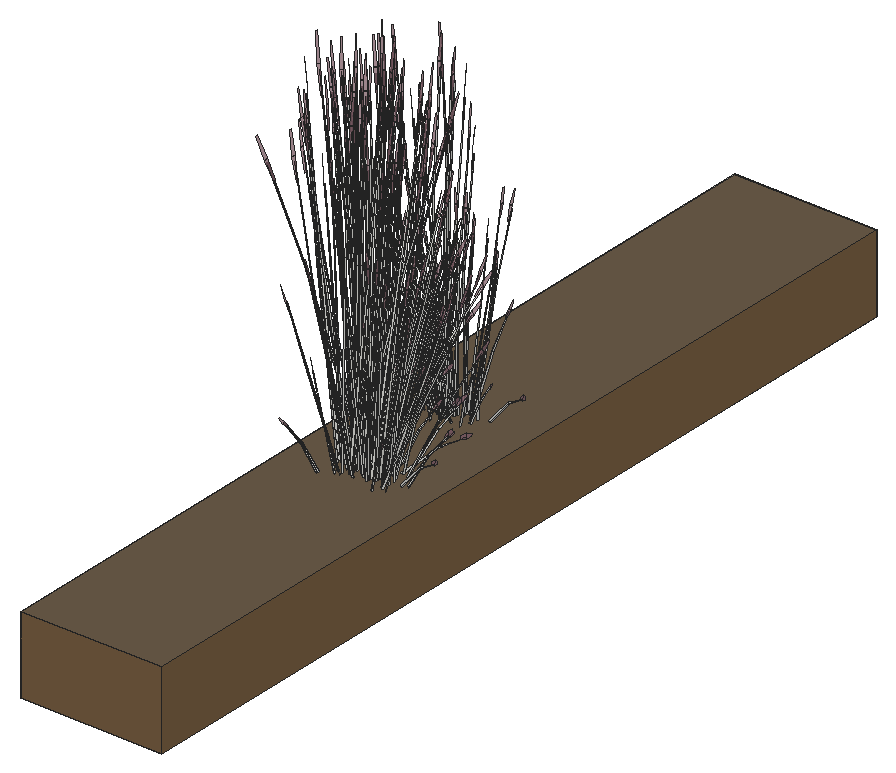
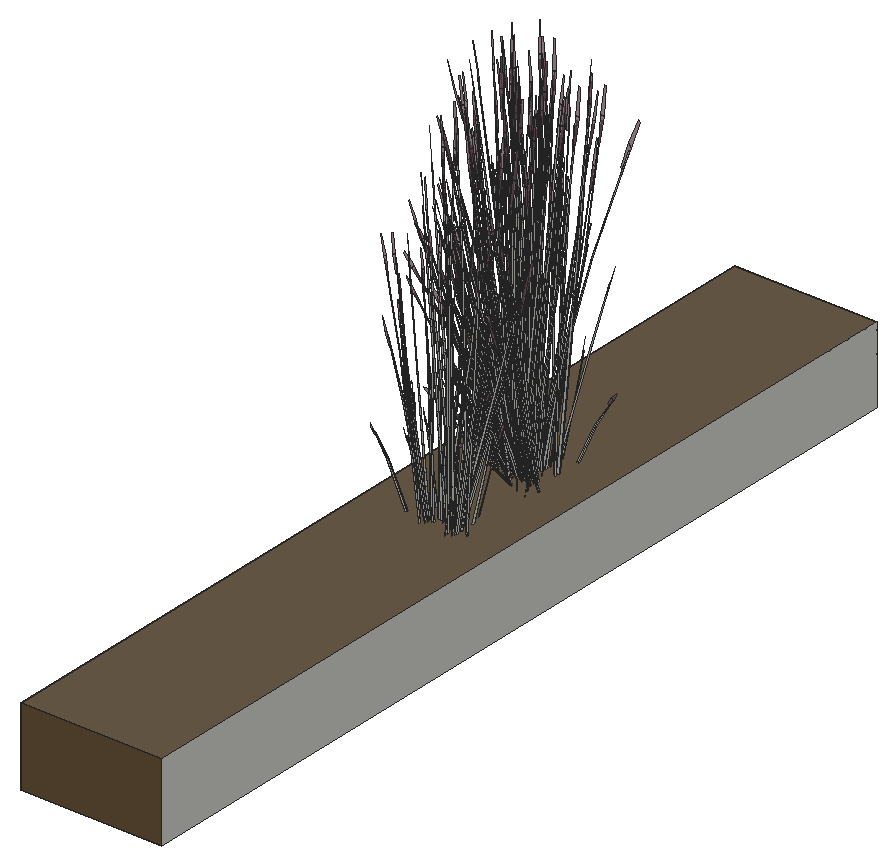
# SketchUp Ruby script. Lengths in inches.
U = 1.inch
M = Sketchup.active_model
def pt(a) = Geom::Point3d.new(a.map { |v| v * U })
def face(e, loops, mat)
  f = e.add_face(loops[0].map { |a| pt(a) })
  loops[1..].each { |l| e.add_face(l.map { |a| pt(a) }).erase! }
  f.material = f.back_material = mat if mat
  f
end
# faces: each face lists its corners as indices into pts; further lists are holes
def faces(e, pts, list, mat = nil) = list.each { |f| face(e, (f[0].is_a?(Array) ? f : [f]).map { |l| l.map { |i| pts[i] } }, mat) }
# xy, xz, yz: faces in a plane at the given z, y or x. An outline is a flat list of corners, or four numbers for a rectangle; further outlines are holes
def ring(l) = l.size == 4 ? [[l[0], l[1]], [l[2], l[1]], [l[2], l[3]], [l[0], l[3]]] : l.each_slice(2).to_a
def flat(e, list, mat, &to3) = list.each { |f| face(e, (f[0].is_a?(Array) ? f : [f]).map { |l| ring(l).map { |u, v| to3.(u, v) } }, mat) }
def xy(e, z, list, mat = nil) = flat(e, list, mat) { |x, y| [x, y, z] }
def xz(e, y, list, mat = nil) = flat(e, list, mat) { |x, z| [x, y, z] }
def yz(e, x, list, mat = nil) = flat(e, list, mat) { |y, z| [x, y, z] }
def lines(e, pts, list) = list.each { |a, b| e.add_line(pt(pts[a]), pt(pts[b])) }
# prism: a flat outline (further loops are holes) pulled along v
def prism(e, loops, v, mat = nil)
  f = face(e, loops, mat); d = Geom::Vector3d.new(v.map { |x| x * U })
  f.pushpull(f.normal.samedirection?(d) ? d.length : -d.length)
end
def box(e, o, s, mat = nil) = prism(e, [[o, [o[0] + s[0], o[1], o[2]], [o[0] + s[0], o[1] + s[1], o[2]], [o[0], o[1] + s[1], o[2]]]], [0, 0, s[2]], mat)
def at(x, y, z, deg = 0) = Geom::Transformation.translation(pt([x, y, z])) * Geom::Transformation.rotation(ORIGIN, Z_AXIS, deg.degrees)
def axes(o, x, y, z) = Geom::Transformation.new([*x, 0, *y, 0, *z, 0, *pt(o).to_a, 1])
def part(name) = M.definitions.add(name)
# library, detail: a bought-in or finely detailed component or shape, given as its bounding box
def library(name, o, s) = part(name).tap { |d| box(d.entities, o, s) }
def detail(e, o, s) = box(e.add_group.entities, o, s)
def put(e, d, t, mat = nil) = e.add_instance(d, t).tap { |i| i.material = mat if mat }
def group(e, t, mat = nil) = e.add_group.tap { |g| g.transformation = t; g.material = mat if mat }.entities
root = M.entities
M.materials.add("Forest_Floor_01_1K").color = [106, 91, 72]
M.materials.add("LightPink_Translucent").color = [144, 107, 117]
M.materials["LightPink_Translucent"].alpha = 0.75
M.materials.add("Soil_03_1K").color = [122, 96, 67]
c1 = part("blade")
p = [[2.15,0.21,22],[0,0.17,0],[0.09,0.45,0],[2.18,0.31,22],[2.29,0.31,22],[0.38,0.45,0],
  [2.48,0.24,33],[2.49,0.24,33],[2.48,0.22,33]]
faces(c1.entities,p,[[0,1,2,3],[4,5,2,3],[6,3,4,7],[8,0,3,6]])
c2 = part("seeds")
p = [[0.3,-0.1,1.38],[-0.01,-0.03,1.59],[-0.01,-0.03,0.03],[0.14,-0.07,-0.07],[0.29,-0.03,3],[0.15,0.01,3.11]]
faces(c2.entities,p,[[0,1,2,3],[1,0,4,5]],"LightPink_Translucent")
c3 = part("blade with seeds")
put(c3.entities,c1,at(0,0,0))
put(c3.entities,c2,axes([2.4,0.25,30.99],[1.5799,-0.05474,1.17369],[-0.12525,1.92788,0.29478],[-0.07173,-0.02425,1.56792]))
xy(root,-6,[[498.15,426.77,519.85,563.22]])
xy(root,5.86,[[498.15,426.77,519.85,563.22]],"Forest_Floor_01_1K")
xz(root,426.77,[[498.15,-6,519.85,5.86]],"Soil_03_1K")
xz(root,563.22,[[498.15,-6,519.85,5.86]],"Soil_03_1K")
yz(root,498.15,[[426.77,-6,563.22,5.86]])
yz(root,519.85,[[426.77,-6,563.22,5.86]],"Soil_03_1K")
put(root,c3,axes([510.03,477.89,3.72],[0.5141,-0.32171,-0.35414],[0.48666,0.36734,0.4572],[0.07405,-0.18664,0.87481]))
put(root,c3,axes([505.58,476.76,1.96],[0.39634,0.21267,1.1486],[-0.57721,0.12784,0.84392],[-0.1235,-0.16344,0.25299]))
put(root,c3,axes([508.52,477.39,3.92],[0.55987,-0.20767,0.0643],[0.27403,0.37869,0.50621],[-0.05407,-0.16693,0.77189]))
put(root,c3,axes([506.61,477.45,3.92],[0.34533,-0.38816,0.0643],[0.49176,0.22599,0.50621],[-0.15898,-0.12445,0.77189]))
put(root,c3,axes([506.5,479.61,1.29],[-0.31203,-0.62659,-0.69835],[0.89884,-0.22566,-0.18329],[-0.03449,-0.21218,1.54149]))
put(root,c3,axes([510.67,477.7,0.6875],[-0.11372,-0.04814,1.76342],[-0.29211,-0.53779,-0.26939],[0.19706,-0.14594,0.30037]))
put(root,c3,axes([508.32,477.82,4.24],[-0.22906,0.4699,0.35414],[-0.66828,-0.13705,-0.4572],[-0.06128,-0.18919,0.87481]))
put(root,c3,axes([510.03,478.02,3.93],[0.54105,0.41691,0.48003],[-0.57458,0.35956,0.3958],[0.0998,-0.1956,0.9933]))
put(root,c3,axes([510.22,478.06,3.92],[0.62439,0.02847,0.0643],[-0.01712,0.42991,0.50621],[0.06534,-0.16468,0.77189]))
put(root,c3,axes([509.76,478.35,4.24],[-0.5141,0.32171,0.35414],[-0.48666,-0.36734,-0.4572],[0.07405,-0.18664,0.87481]))
put(root,c3,axes([510.67,479.22,4.17],[0.39688,-0.48213,-0.71045],[0.69548,0.34264,0.08574],[0.23697,-0.17468,1.00501]))
put(root,c3,axes([506.375,477.8125,1.57],[-0.47504,-0.61229,0],[0.79476,-0.34146,-0.51607],[0.18101,-0.07777,1.63711]))
put(root,c3,axes([510.65,478.99,3.875],[-0.19519,-0.55794,-0.51099],[0.73919,-0.0976,-0.3958],[0.21183,-0.14986,0.97773]))
put(root,c3,axes([507.42,477.07,1.32],[-0.52505,0.35054,-0.03893],[-0.48109,-0.38392,-0.17649],[-0.03387,-0.10878,0.58215]))
put(root,c3,axes([510.99,479.39,4.23],[-0.70283,-0.33692,-0.1216],[0.40491,-0.48793,-0.67495],[0.19857,-0.16961,1.02557]))
put(root,c3,axes([508.09,481.23,2.52],[0.65659,0.2464,1.51261],[-0.64324,0.53082,0.59816],[-0.28812,-0.31461,1.26806]))
put(root,c3,axes([504.66,479.53,1.21],[0,-0.61104,-0.49651],[0.85008,0,0],[0,-0.13917,1.57504]))
put(root,c3,axes([507.02,477.72,1.21],[0.7111,-0.30552,-0.49651],[0.42504,0.54784,0],[0.16196,-0.06958,1.57504]))
put(root,c3,axes([511.24,478.77,1.78],[-0.27143,-0.0181,1.43002],[-0.27808,-0.48551,-0.30754],[0.33346,-0.13735,0.61141]))
put(root,c3,axes([512.72,479.24,3.9],[-0.09924,-0.00464,1.77383],[-0.4121,-0.49725,-0.16761],[0.1655,-0.1635,0.31391]))
put(root,c3,axes([507.86,478.97,1.25],[0.51177,-0.45928,-0.62353],[0.63575,0.41646,-0.16365],[0.20507,-0.11457,1.37633]))
put(root,c3,axes([511.55,477.88,1.96],[-0.25308,0.31105,1.1486],[-0.21753,-0.4179,0.84392],[0.20902,-0.10472,0.25299]))
put(root,c3,axes([511.19,479.05,3.72],[0.66138,-0.08733,-0.35414],[0.17464,0.49921,0.4572],[0.18953,-0.13408,0.87481]))
put(root,c3,axes([506.97,479.78,1.4],[0.36864,-0.55059,-0.44739],[0.76598,0.26498,0.21531],[0,-0.12692,1.43643]))
put(root,c3,axes([507.31,479.5,1.86],[-0.08854,-0.69723,-0.29095],[0.92215,-0.04216,-0.50002],[0.16238,-0.09287,1.59708]))
put(root,c3,axes([505.02,479.54,1.22],[0.53038,-0.38124,-0.30978],[0.53038,0.38124,0.30978],[0,-0.1228,1.38974]))
put(root,c3,axes([510.65,479.34,4.24],[-0.66138,0.08733,0.35414],[-0.17464,-0.49921,-0.4572],[0.18953,-0.13408,0.87481]))
put(root,c3,axes([506.88,480.23,1.86],[-0.85568,-0.29155,-0.29095],[0.41201,-0.61537,-0.50002],[-0.02689,-0.15109,1.59708]))
put(root,c3,axes([507.1875,477.96,1.22],[0.70886,0.15119,-0.30978],[-0.17848,0.53243,0.30978],[0.1429,-0.0614,1.38974]))
put(root,c3,axes([511.25,479.27,3.92],[0.52161,0.25698,0.0643],[-0.30368,0.36595,0.50621],[0.16723,-0.11831,0.77189]))
put(root,c3,axes([511.11,479.16,3.93],[0.18844,0.56237,0.48003],[-0.73919,0.0976,0.3958],[0.21785,-0.13226,0.9933]))
put(root,c3,axes([513.1,479.84,3.91],[0.10543,-0.09307,1.74944],[-0.13495,-0.57092,-0.27667],[0.26455,-0.10825,0.14031]))
put(root,c3,axes([505.18,479.81,1.52],[-0.70674,0.51372,0.30756],[-0.70717,-0.50832,-0.36492],[-0.02468,-0.14589,1.64885]))
put(root,c3,axes([507.43,480.05,1.625],[0.8561,0.29616,0.24065],[-0.41201,0.61537,0.50002],[0,-0.14185,1.60543]))
put(root,c3,axes([507.1,480.88,1.63],[0.20138,-0.72405,-0.23429],[0.95485,0.12621,0.51271],[-0.16685,-0.09999,1.5644]))
put(root,c3,axes([507.15,479.64,1.91],[-0.82508,0.03772,0.44739],[-0.07462,-0.62614,-0.21531],[0.14771,-0.06346,1.43643]))
put(root,c3,axes([505.02,480.09,1.67],[0,0.61104,0.49651],[-0.85008,0,0],[0,-0.13917,1.57504]))
put(root,c3,axes([511.02,480.71,4.23],[-0.38229,-0.5533,-0.1216],[0.6785,-0.2719,-0.67495],[0.28593,-0.073,1.02557]))
put(root,c3,axes([510.99,480.23,3.875],[0.20584,-0.55581,-0.51099],[0.70573,0.19051,-0.3958],[0.28414,-0.05097,0.97773]))
put(root,c3,axes([509.875,477.97,1.57],[0.47504,-0.61229,0],[0.79476,0.34146,-0.51607],[0.18101,0.07777,1.63711]))
put(root,c3,axes([507.03,480.59,1.4],[-0.45644,-0.51287,-0.44739],[0.69137,-0.36116,0.21531],[-0.14771,-0.06346,1.43643]))
put(root,c3,axes([507.125,479.86,1.55],[0.33034,0.68327,0.45755],[-0.94388,0.2376,0.17955],[0.01154,-0.12555,1.58856]))
put(root,c3,axes([511.74,480.39,1.17],[-0.48937,0.07333,1.41583],[-0.07789,-0.58369,0.08104],[0.34275,-0.08835,0.80566]))
put(root,c3,axes([512.63,479.87,1.45],[-0.47106,-0.39072,-0.06488],[0.51591,-0.35801,-0.29416],[0.14618,-0.02521,0.97024]))
put(root,c3,axes([506.96,480.4,1.91],[-0.36864,0.55059,0.44739],[-0.76598,-0.26498,-0.21531],[0,-0.12692,1.43643]))
put(root,c3,axes([508.3125,479.92,1.4],[0,-0.70701,0],[0.95008,0,0],[0,0,1.79456]))
put(root,c3,axes([509.46,478.29,1.67],[-0.7111,-0.30552,0.49651],[0.42504,-0.54784,0],[0.16196,0.06958,1.57504]))
put(root,c3,axes([510.85,480.43,4.17],[0.66765,-0.26986,-0.71045],[0.37208,0.55551,0.08574],[0.32259,-0.0631,1.00501]))
put(root,c3,axes([507.86,479.47,1.55],[-0.62999,0.55453,0.45755],[-0.74845,-0.4895,0.17955],[0.15188,-0.05534,1.58856]))
put(root,c3,axes([508.55,480.47,1.49],[-0.70674,-0.52593,-0.06131],[0.70717,-0.52625,0],[-0.02468,-0.01837,1.75571]))
put(root,c3,axes([506.77,478.5625,1.67],[-0.21949,0.60727,0.17642],[-0.8032,-0.17185,0.35086],[0.13875,-0.00296,1.60407]))
put(root,c3,axes([510.76,480.54,4.24],[-0.63144,-0.17046,0.35414],[0.18417,-0.49731,-0.4572],[0.25423,-0.0456,0.87481]))
put(root,c3,axes([506.4375,479.05,0.79],[-0.74787,0.24464,1.28929],[-0.23804,-0.70192,0.50096],[0.45924,0.01168,1.46642]))
put(root,c3,axes([508.45,479.24,1.81],[0.14658,-0.54532,0.1448],[0.71613,0.09466,-0.41347],[0.13033,0.05599,1.26744]))
put(root,c3,axes([507.21,480.53,1.55],[0.96033,0.12874,0.45755],[-0.19544,0.7271,0.17955],[-0.14034,-0.07021,1.58856]))
put(root,c3,axes([512.28,480.01,0.6875],[-0.03971,-0.09277,1.76342],[0.27541,-0.54264,-0.26939],[0.27782,-0.00781,0.30037]))
put(root,c3,axes([508.14,479.38,1.91],[-0.45644,-0.51287,0.44739],[0.69137,-0.36116,-0.21531],[0.14771,0.06346,1.43643]))
put(root,c3,axes([506.69,481.69,1.67],[0.81646,-0.16218,0.17642],[0.20161,0.60355,0.35086],[-0.07282,-0.08794,1.60407]))
put(root,c3,axes([508.37,479.41,1.86],[0.76714,-0.40567,-0.29095],[0.51013,0.57321,-0.50002],[0.18927,0.05821,1.59708]))
put(root,c3,axes([511.42,480.48,3.72],[0.63144,0.17046,-0.35414],[-0.18417,0.49731,0.4572],[0.25423,-0.0456,0.87481]))
put(root,c3,axes([510.31,478.34,1.21],[0.7111,0.30552,-0.49651],[-0.42504,0.54784,0],[0.16196,0.06958,1.57504]))
put(root,c3,axes([508.96,480.08,1.4],[0.85008,0,0],[0,0.63259,0],[0,0,1.78407]))
put(root,c3,axes([509.2,478.59,1.67],[-0.81646,0.16218,0.17642],[-0.20161,-0.60355,0.35086],[0.07282,0.08794,1.60407]))
put(root,c3,axes([509.7,479.87,3.07],[-0.31515,0.01384,1.71376],[0.20907,-0.5998,0.13857],[0.44912,0.0371,0.73262]))
put(root,c3,axes([510.11,478.5625,1.22],[0.17848,0.53243,-0.30978],[-0.70886,0.15119,0.30978],[0.1429,0.0614,1.38974]))
put(root,c3,axes([511.33,480.69,3.92],[0.27906,0.41663,0.0643],[-0.50888,0.20393,0.50621],[0.22432,-0.04024,0.77189]))
put(root,c3,axes([508.68,479.76,1.57],[-0.96033,-0.12874,0.49198],[0.19544,-0.7271,0.19306],[0.14034,0.07021,1.70813]))
put(root,c3,axes([511.28,480.55,3.93],[-0.21466,0.55714,0.48003],[-0.70573,-0.19051,0.3958],[0.27753,-0.03348,0.9933]))
put(root,c3,axes([507.92,481.55,1.4],[-0.24791,-0.5268,0],[0.70791,-0.18448,0],[0,0,1.54371]))
put(root,c3,axes([507.44,481.05,1.81],[-0.14658,0.54532,0.1448],[-0.71613,-0.09466,-0.41347],[-0.13033,-0.05599,1.26744]))
put(root,c3,axes([508.84,481.48,1.38],[0.79769,-0.20732,-0.19198],[0.2803,0.59721,0.00008],[0.08805,-0.02292,1.73897]))
put(root,c3,axes([509.12,481.73,1.67],[0.21949,-0.60727,0.17642],[0.8032,0.17185,0.35086],[-0.13875,0.00296,1.60407]))
put(root,c3,axes([508.9375,480.35,1.41],[0.53038,0.39469,0],[-0.53038,0.39469,0],[0,0,1.69266]))
put(root,c3,axes([510.375,480.18,1.67],[-0.59697,-0.44509,0.17642],[0.60159,-0.4317,0.35086],[-0.06593,0.0909,1.60407]))
put(root,c3,axes([509.27,479.51,1.25],[0.79037,0.10018,-0.62353],[-0.16679,0.61794,-0.16365],[0.23587,0.07488,1.37633]))
put(root,c3,axes([512.76,480.58,1.96],[-0.46945,0.10088,1.1486],[0.22097,-0.4169,0.84392],[0.24904,0.02853,0.25299]))
put(root,c3,axes([507.74,481.79,1.39],[-0.76598,-0.27433,0],[0.36864,-0.57001,0],[0,0,1.62707]))
put(root,c3,axes([508.38,481.06,1.66],[-0.74193,-0.49181,-0.25192],[0.6243,-0.55226,0.5513],[-0.19979,0.05753,1.68216]))
put(root,c3,axes([506.42,482,1.67],[0.7111,0.30552,0.49651],[-0.42504,0.54784,0],[-0.16196,-0.06958,1.57504]))
put(root,c3,axes([508.93,479.89,1.91],[0.36864,-0.55059,0.44739],[0.76598,0.26498,-0.21531],[0,0.12692,1.43643]))
put(root,c3,axes([512.54,482.35,3.9],[-0.0687,-0.05349,1.77383],[0.15029,-0.57341,-0.16761],[0.27062,-0.03664,0.31391]))
put(root,c3,axes([508.79,480.2,1.48],[0,0.70667,-0.05637],[-0.95008,0,0],[0,0.02221,1.79368]))
put(root,c3,axes([508.86,479.7,1.4],[0.45644,0.51287,-0.44739],[-0.69137,0.36116,0.21531],[0.14771,0.06346,1.43643]))
put(root,c3,axes([511.95,481.87,3.12],[-0.14542,-0.51365,-0.03492],[0.68734,-0.11809,-0.15832],[0.14353,0.03256,0.52218]))
put(root,c3,axes([510.16,481.85,4.23],[0.04068,-0.62141,-0.1216],[0.77029,0.01698,-0.67495],[0.29667,0.04317,1.02557]))
put(root,c3,axes([510.87,480.19,1.67],[0,-0.61104,0.49651],[0.85008,0,0],[0,0.13917,1.57504]))
put(root,c3,axes([508.74,480.65,1.91],[0.82508,-0.03772,0.44739],[0.07462,0.62614,-0.21531],[-0.14771,0.06346,1.43643]))
put(root,c3,axes([509.25,480.01,1.81],[0.70791,-0.1782,0.1448],[0.24791,0.50885,-0.41347],[0,0.11199,1.26744]))
put(root,c3,axes([510.05,481.61,4.24],[-0.43232,-0.38257,0.35414],[0.49364,-0.36215,-0.4572],[0.25081,0.0551,0.87481]))
put(root,c3,axes([508,480.96,1.4],[-0.82508,0.03772,-0.44739],[-0.07462,-0.62614,0.21531],[-0.14771,0.06346,1.43643]))
put(root,c3,axes([511.88,481.25,1.78],[-0.18299,-0.15028,1.43002],[0.23809,-0.49714,-0.30754],[0.37023,0.06735,0.61141]))
put(root,c3,axes([508.61,481.8,1.4],[0.76598,0.27433,0],[-0.36864,0.57001,0],[0,0,1.74954]))
put(root,c3,axes([510.83,481.48,3.91],[0.16299,-0.01033,1.74944],[0.44707,-0.47471,-0.27667],[0.28992,0.06266,0.14031]))
put(root,c3,axes([508.92,482.41,1.39],[-0.46912,-0.61443,-0.05142],[0.79476,-0.34146,0.51607],[-0.19584,0.0585,1.6363]))
put(root,c3,axes([508.75,480.92,1.81],[0.56134,0.36712,0.1448],[-0.46823,0.41419,-0.41347],[-0.13033,0.05599,1.26744]))
put(root,c3,axes([510.2,481.56,4.17],[0.75952,0.01471,-0.71045],[-0.05101,0.61953,0.08574],[0.32177,0.06538,1.00501]))
put(root,c3,axes([509.35,482.05,1.67],[0.7111,-0.30552,0.49651],[0.42504,0.54784,0],[-0.16196,0.06958,1.57504]))
put(root,c3,axes([508.34,481.57,1.48],[0.33034,0.70197,-0.06012],[-0.94388,0.24598,0],[0.01154,0.02451,1.72173]))
put(root,c3,axes([508.7,482.33,1.22],[-0.70886,-0.15119,-0.30978],[0.17848,-0.53243,0.30978],[-0.1429,0.0614,1.38974]))
put(root,c3,axes([511.44,480.3,1.57],[0.95008,0,0],[0,0.68292,-0.51607],[0,0.15554,1.63711]))
put(root,c3,axes([511.0625,480.65,1.39],[-0.94962,-0.00489,-0.04976],[0,-0.68292,0.49943],[-0.02984,0.15546,1.58352]))
put(root,c3,axes([509.01,480.06,1.86],[0.85568,0.29155,-0.29095],[-0.41201,0.61537,-0.50002],[0.02689,0.15109,1.59708]))
put(root,c3,axes([510.66,481.8125,3.72],[0.43232,0.38257,-0.35414],[-0.49364,0.36215,0.4572],[0.25081,0.0551,0.87481]))
put(root,c3,axes([510.87,480.75,1.22],[-0.53038,0.38124,-0.30978],[-0.53038,-0.38124,0.30978],[0,0.1228,1.38974]))
put(root,c3,axes([508.58,480.79,1.86],[0.08854,0.69723,-0.29095],[-0.92215,0.04216,-0.50002],[-0.16238,0.09287,1.59708]))
put(root,c3,axes([510.4375,481.96,3.92],[-0.03826,0.46465,0.0643],[-0.57772,-0.01274,0.50621],[0.2213,0.04862,0.77189]))
put(root,c3,axes([508.92,480.51,1.4],[-0.36864,0.55059,-0.44739],[-0.76598,-0.26498,0.21531],[0,0.12692,1.43643]))
put(root,c3,axes([510.49,481.81,3.93],[-0.56024,0.40262,0.48003],[-0.48318,-0.42758,0.3958],[0.26285,0.07427,0.9933]))
put(root,c3,axes([508.71,482.28,4.24],[-0.11735,-0.49217,0.35414],[0.67083,-0.12996,-0.4572],[0.18018,0.14104,0.87481]))
put(root,c3,axes([508.9375,482.09,1.52],[0.95122,0.19861,0.30756],[-0.23797,0.7099,-0.36492],[-0.15744,0.08885,1.64885]))
put(root,c3,axes([508.87,482.57,1.21],[-0.7111,0.30552,-0.49651],[-0.42504,-0.54784,0],[-0.16196,0.06958,1.57504]))
put(root,c3,axes([511.23,480.76,1.21],[0,0.61104,-0.49651],[-0.85008,0,0],[0,0.13917,1.57504]))
put(root,c3,axes([509.11,480.83,3.07],[-0.28223,-0.10528,1.71376],[0.58406,-0.44165,0.13857],[0.36402,0.19924,0.73262]))
put(root,c3,axes([509.16,479.44,3.67],[-0.65655,-0.31748,1.38283],[0.69326,-0.49431,0.59665],[0.21183,0.29789,1.33663]))
put(root,c3,axes([510.15,482.03,1.96],[-0.4278,-0.1757,1.1486],[0.5524,-0.17852,0.84392],[0.14899,0.15122,0.25299]))
put(root,c3,axes([508.65,482.53,4.23],[0.45276,-0.52302,-0.1216],[0.65568,0.30132,-0.67495],[0.22792,0.14777,1.02557]))
put(root,c3,axes([505.66,481.82,4.24],[0.5141,-0.32171,0.35414],[0.48666,0.36734,-0.4572],[-0.07405,0.18664,0.87481]))
put(root,c3,axes([509.51,482.48,1.57],[0.47504,0.61229,0],[-0.79476,0.34146,-0.51607],[-0.18101,0.07777,1.63711]))
put(root,c3,axes([508.06,482.96,3.9],[0.00225,-0.07398,1.77383],[0.65113,-0.32638,-0.16761],[0.22617,0.1165,0.31391]))
put(root,c3,axes([510.27,482.68,0.6875],[0.05536,-0.08822,1.76342],[0.69692,-0.25981,-0.26939],[0.21129,0.13447,0.30037]))
put(root,c3,axes([509.11,480.05,2.03],[-0.02076,-0.57531,1.41272],[0.93937,0.14913,0.59816],[-0.22217,0.31481,1.3335]))
put(root,c3,axes([509.35,480.68,1.29],[0.2786,0.55945,-0.69212],[-0.80253,0.20149,-0.18165],[0.03079,0.18945,1.52773]))
put(root,c3,axes([509.18,482.27,3.875],[0.74975,-0.14525,-0.51099],[0.13115,0.55007,-0.3958],[0.20138,0.15763,0.97773]))
put(root,c3,axes([507.1,482.35,4.24],[0.22906,-0.4699,0.35414],[0.66828,0.13705,-0.4572],[0.06128,0.18919,0.87481]))
put(root,c3,axes([510.22,482.83,1.86],[-0.48723,-0.01916,1.0506],[0.32177,-0.40701,0.58006],[0.19248,0.1446,0.8241]))
put(root,c3,axes([508.82,482.72,3.92],[-0.34533,0.38816,0.0643],[-0.49176,-0.22599,0.50621],[0.15898,0.12445,0.77189]))
put(root,c3,axes([508,484.03,4.84],[0.52505,-0.35054,-0.06488],[0.48109,0.38392,-0.29416],[0.03387,0.10878,0.97024]))
put(root,c3,axes([508.96,482.61,3.93],[-0.75571,0.14023,0.48003],[-0.13115,-0.55007,0.3958],[0.17773,0.16212,0.9933]))
put(root,c3,axes([508.63,481.84,1.78],[0.01341,-0.20255,1.43002],[0.64074,-0.22625,-0.30754],[0.1978,0.24243,0.61141]))
put(root,c3,axes([506.9,482.78,3.92],[-0.55987,0.20767,0.0643],[-0.27403,-0.37869,0.50621],[0.05407,0.16693,0.77189]))
put(root,c3,axes([505.34,481.91,4.59],[0.83505,0.03027,-0.13498],[-0.02282,0.57322,-0.74919],[-0.05801,0.22077,1.13838]))
put(root,c3,axes([506.88,482.55,4.23],[0.74352,-0.28449,-0.1216],[0.36538,0.50492,-0.67495],[0.0981,0.21277,1.02557]))
put(root,c3,axes([507.1,482.74,4.26],[-0.74868,-0.15974,0.53283],[0.25601,-0.52518,0.43934],[0.04499,0.20653,1.10256]))
put(root,c3,axes([505.72,483.53,1.96],[-0.01966,-0.36332,1.1486],[0.49135,0.25914,0.84392],[-0.09663,0.17317,0.25299]))
put(root,c3,axes([507.02,482.66,0.6875],[0.12297,-0.03325,1.76342],[0.73967,0.18301,-0.26939],[0.02163,0.20626,0.30037]))
put(root,c3,axes([505.91,482.13,4.2],[0.54391,0.41056,-0.5672],[-0.57458,0.35956,-0.43934],[-0.08276,0.2086,1.08528]))
put(root,c3,axes([505.32,482.75,2.02],[0.69024,-0.1082,0.06507],[0.15868,0.43593,-0.86304],[-0.04376,0.22067,0.7736]))
put(root,c3,axes([507.52,482.53,3.875],[0.7469,0.15318,-0.51099],[-0.25601,0.52518,-0.3958],[0.06849,0.21144,0.97773]))
put(root,c3,axes([507.94,481.44,3.07],[-0.17368,-0.19618,1.71376],[0.80256,-0.16516,0.13857],[0.18139,0.30799,0.73262]))
put(root,c3,axes([507.18,482.85,3.72],[-0.22906,0.4699,-0.35414],[-0.66828,-0.13705,0.4572],[0.06128,0.18919,0.87481]))
put(root,c3,axes([505.74,481.94,4.53],[-0.01977,0.56521,-0.7886],[-0.83252,-0.03796,0.09517],[-0.08786,0.23945,1.11556]))
put(root,c3,axes([503.5625,483.43,3.9],[0.0862,-0.03689,1.77383],[0.71245,0.24539,-0.16761],[-0.01674,0.20431,0.31391]))
put(root,c3,axes([506.52,481.54,3.07],[-0.0186,-0.23452,1.71376],[0.80601,0.15558,0.13857],[-0.04985,0.33422,0.73262]))
put(root,c3,axes([507.25,482.43,4.17],[0.36264,0.49684,-0.71045],[-0.74649,0.27689,0.08574],[0.0848,0.24006,1.00501]))
put(root,c3,axes([506.71,483.68,3.91],[0.09631,0.0984,1.74944],[0.77725,0.03866,-0.27667],[0.07816,0.217,0.14031]))
put(root,c3,axes([505.46,482.74,2.56],[0.01669,-0.31544,1.54345],[0.75083,0.16661,0.21329],[-0.06506,0.33618,0.72882]))
put(root,c3,axes([507.52,496.24,1.78],[-0.21597,0.12368,1.43002],[-0.64681,-0.21647,-0.30754],[0.1199,-0.26922,0.61141]))
put(root,c3,axes([506.54,496.67,4.17],[-0.36264,-0.49684,-0.71045],[0.74649,-0.27689,0.08574],[-0.0848,-0.24006,1.00501]))
put(root,c3,axes([505.91,495.57,0.6875],[-0.12744,0.02202,1.76342],[-0.70477,-0.24781,-0.26939],[0.01183,-0.2067,0.30037]))
put(root,c3,axes([508.05,497.15,4.17],[0.01977,-0.56521,-0.71045],[0.83252,0.03796,0.08574],[0.08786,-0.23945,1.00501]))
put(root,c3,axes([509.21,496.27,3.91],[-0.00733,-0.12161,1.74944],[-0.61946,-0.35147,-0.27667],[0.09577,-0.21306,0.14031]))
put(root,c3,axes([506.61,496.25,3.72],[0.22906,-0.4699,-0.35414],[0.66828,0.13705,0.4572],[-0.06128,-0.18919,0.87481]))
put(root,c3,axes([507.11,496.87,3.07],[-0.14147,0.21002,1.71376],[-0.59349,-0.43464,0.13857],[0.26773,-0.27089,0.73262]))
put(root,c3,axes([509.04,495.83,3.9],[-0.07716,0.04667,1.77383],[-0.75601,-0.15746,-0.16761],[-0.02737,-0.20368,0.31391]))
put(root,c3,axes([506.26,496.57,3.875],[-0.7469,-0.15318,-0.51099],[0.25601,-0.52518,-0.3958],[-0.06849,-0.21144,0.97773]))
put(root,c3,axes([506.73,495.25,1.96],[0.09747,0.35631,1.1486],[-0.54071,-0.19735,0.84392],[0.05818,-0.18244,0.25299]))
put(root,c3,axes([507.88,496.97,3.875],[-0.54391,-0.41056,-0.51099],[0.57458,-0.35956,-0.3958],[0.08276,-0.2086,0.97773]))
put(root,c3,axes([506.6875,496.35,3.93],[0.74868,0.15974,0.48003],[-0.25601,0.52518,0.3958],[-0.04499,-0.20653,0.9933]))
put(root,c3,axes([506.9,496.54,4.23],[-0.74352,0.28449,-0.1216],[-0.36538,-0.50492,-0.67495],[-0.0981,-0.21277,1.02557]))
put(root,c3,axes([508.45,497.18,4.23],[-0.83505,-0.03027,-0.1216],[0.02282,-0.57322,-0.67495],[0.05801,-0.22077,1.02557]))
put(root,c3,axes([508.39,496.8125,3.72],[0.5141,-0.32171,-0.35414],[0.48666,0.36734,0.4572],[0.07405,-0.18664,0.87481]))
put(root,c3,axes([506.89,496.31,3.92],[0.55987,-0.20767,0.0643],[0.27403,0.37869,0.50621],[-0.05407,-0.16693,0.77189]))
put(root,c3,axes([504.86,498.53,1.29],[-0.31203,-0.62659,-0.69835],[0.89884,-0.22566,-0.18329],[-0.03449,-0.21218,1.54149]))
put(root,c3,axes([509.03,496.62,0.6875],[-0.11372,-0.04814,1.76342],[-0.29211,-0.53779,-0.26939],[0.19706,-0.14594,0.30037]))
put(root,c3,axes([506.68,496.74,4.24],[-0.22906,0.4699,0.35414],[-0.66828,-0.13705,-0.4572],[-0.06128,-0.18919,0.87481]))
put(root,c3,axes([508.39,496.9375,3.93],[0.54105,0.41691,0.48003],[-0.57458,0.35956,0.3958],[0.0998,-0.1956,0.9933]))
put(root,c3,axes([508.59,496.98,3.92],[0.62439,0.02847,0.0643],[-0.01712,0.42991,0.50621],[0.06534,-0.16468,0.77189]))
put(root,c3,axes([508.12,497.27,4.24],[-0.5141,0.32171,0.35414],[-0.48666,-0.36734,-0.4572],[0.07405,-0.18664,0.87481]))
put(root,c3,axes([509.03,498.14,4.17],[0.39688,-0.48213,-0.71045],[0.69548,0.34264,0.08574],[0.23697,-0.17468,1.00501]))
put(root,c3,axes([504.74,496.73,1.57],[-0.47504,-0.61229,0],[0.79476,-0.34146,-0.51607],[0.18101,-0.07777,1.63711]))
put(root,c3,axes([509.01,497.91,3.875],[-0.19519,-0.55794,-0.51099],[0.73919,-0.0976,-0.3958],[0.21183,-0.14986,0.97773]))
put(root,c3,axes([505.78,495.99,1.32],[-0.52505,0.35054,-0.03893],[-0.48109,-0.38392,-0.17649],[-0.03387,-0.10878,0.58215]))
put(root,c3,axes([509.36,498.31,4.23],[-0.70283,-0.33692,-0.1216],[0.40491,-0.48793,-0.67495],[0.19857,-0.16961,1.02557]))
put(root,c3,axes([505.38,496.64,1.21],[0.7111,-0.30552,-0.49651],[0.42504,0.54784,0],[0.16196,-0.06958,1.57504]))
put(root,c3,axes([509.6,497.69,1.78],[-0.27143,-0.0181,1.43002],[-0.27808,-0.48551,-0.30754],[0.33346,-0.13735,0.61141]))
put(root,c3,axes([511.09,498.16,3.9],[-0.09924,-0.00464,1.77383],[-0.4121,-0.49725,-0.16761],[0.1655,-0.1635,0.31391]))
put(root,c3,axes([506.23,497.89,1.25],[0.51177,-0.45928,-0.62353],[0.63575,0.41646,-0.16365],[0.20507,-0.11457,1.37633]))
put(root,c3,axes([509.92,496.8,1.96],[-0.25308,0.31105,1.1486],[-0.21753,-0.4179,0.84392],[0.20902,-0.10472,0.25299]))
put(root,c3,axes([509.55,497.97,3.72],[0.66138,-0.08733,-0.35414],[0.17464,0.49921,0.4572],[0.18953,-0.13408,0.87481]))
put(root,c3,axes([505.33,498.7,1.4],[0.36864,-0.55059,-0.44739],[0.76598,0.26498,0.21531],[0,-0.12692,1.43643]))
put(root,c3,axes([505.67,498.42,1.86],[-0.08854,-0.69723,-0.29095],[0.92215,-0.04216,-0.50002],[0.16238,-0.09287,1.59708]))
put(root,c3,axes([503.38,498.46,1.22],[0.53038,-0.38124,-0.30978],[0.53038,0.38124,0.30978],[0,-0.1228,1.38974]))
put(root,c3,axes([509.01,498.26,4.24],[-0.66138,0.08733,0.35414],[-0.17464,-0.49921,-0.4572],[0.18953,-0.13408,0.87481]))
put(root,c3,axes([505.24,499.15,1.86],[-0.85568,-0.29155,-0.29095],[0.41201,-0.61537,-0.50002],[-0.02689,-0.15109,1.59708]))
put(root,c3,axes([505.55,496.88,1.22],[0.70886,0.15119,-0.30978],[-0.17848,0.53243,0.30978],[0.1429,-0.0614,1.38974]))
put(root,c3,axes([509.61,498.19,3.92],[0.52161,0.25698,0.0643],[-0.30368,0.36595,0.50621],[0.16723,-0.11831,0.77189]))
put(root,c3,axes([509.47,498.08,3.93],[0.18844,0.56237,0.48003],[-0.73919,0.0976,0.3958],[0.21785,-0.13226,0.9933]))
put(root,c3,axes([511.46,498.76,3.91],[0.10543,-0.09307,1.74944],[-0.13495,-0.57092,-0.27667],[0.26455,-0.10825,0.14031]))
put(root,c3,axes([505.79,498.97,1.625],[0.8561,0.29616,0.24065],[-0.41201,0.61537,0.50002],[0,-0.14185,1.60543]))
put(root,c3,axes([505.51,498.56,1.91],[-0.82508,0.03772,0.44739],[-0.07462,-0.62614,-0.21531],[0.14771,-0.06346,1.43643]))
put(root,c3,axes([509.39,499.625,4.23],[-0.38229,-0.5533,-0.1216],[0.6785,-0.2719,-0.67495],[0.28593,-0.073,1.02557]))
